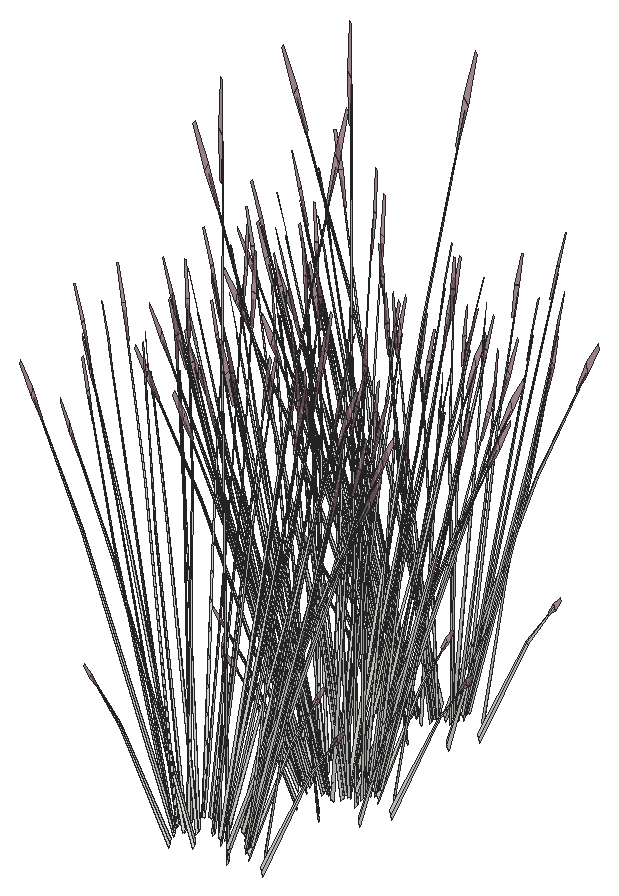
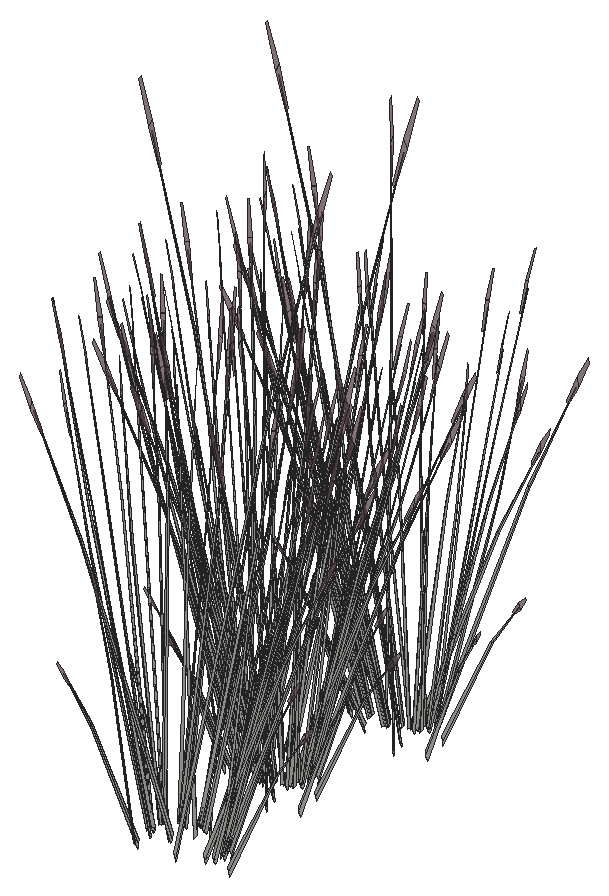
# SketchUp Ruby script. Lengths in inches.
U = 1.inch
M = Sketchup.active_model
def pt(a) = Geom::Point3d.new(a.map { |v| v * U })
def face(e, loops, mat)
  f = e.add_face(loops[0].map { |a| pt(a) })
  loops[1..].each { |l| e.add_face(l.map { |a| pt(a) }).erase! }
  f.material = f.back_material = mat if mat
  f
end
# faces: each face lists its corners as indices into pts; further lists are holes
def faces(e, pts, list, mat = nil) = list.each { |f| face(e, (f[0].is_a?(Array) ? f : [f]).map { |l| l.map { |i| pts[i] } }, mat) }
# xy, xz, yz: faces in a plane at the given z, y or x. An outline is a flat list of corners, or four numbers for a rectangle; further outlines are holes
def ring(l) = l.size == 4 ? [[l[0], l[1]], [l[2], l[1]], [l[2], l[3]], [l[0], l[3]]] : l.each_slice(2).to_a
def flat(e, list, mat, &to3) = list.each { |f| face(e, (f[0].is_a?(Array) ? f : [f]).map { |l| ring(l).map { |u, v| to3.(u, v) } }, mat) }
def xy(e, z, list, mat = nil) = flat(e, list, mat) { |x, y| [x, y, z] }
def xz(e, y, list, mat = nil) = flat(e, list, mat) { |x, z| [x, y, z] }
def yz(e, x, list, mat = nil) = flat(e, list, mat) { |y, z| [x, y, z] }
def lines(e, pts, list) = list.each { |a, b| e.add_line(pt(pts[a]), pt(pts[b])) }
# prism: a flat outline (further loops are holes) pulled along v
def prism(e, loops, v, mat = nil)
  f = face(e, loops, mat); d = Geom::Vector3d.new(v.map { |x| x * U })
  f.pushpull(f.normal.samedirection?(d) ? d.length : -d.length)
end
def box(e, o, s, mat = nil) = prism(e, [[o, [o[0] + s[0], o[1], o[2]], [o[0] + s[0], o[1] + s[1], o[2]], [o[0], o[1] + s[1], o[2]]]], [0, 0, s[2]], mat)
def at(x, y, z, deg = 0) = Geom::Transformation.translation(pt([x, y, z])) * Geom::Transformation.rotation(ORIGIN, Z_AXIS, deg.degrees)
def axes(o, x, y, z) = Geom::Transformation.new([*x, 0, *y, 0, *z, 0, *pt(o).to_a, 1])
def part(name) = M.definitions.add(name)
# library, detail: a bought-in or finely detailed component or shape, given as its bounding box
def library(name, o, s) = part(name).tap { |d| box(d.entities, o, s) }
def detail(e, o, s) = box(e.add_group.entities, o, s)
def put(e, d, t, mat = nil) = e.add_instance(d, t).tap { |i| i.material = mat if mat }
def group(e, t, mat = nil) = e.add_group.tap { |g| g.transformation = t; g.material = mat if mat }.entities
root = M.entities
M.materials.add("LightPink_Translucent").color = [144, 107, 117]
M.materials["LightPink_Translucent"].alpha = 0.75
c1 = part("blade")
p = [[2.15,0.21,22],[0,0.17,0],[0.09,0.45,0],[2.18,0.31,22],[2.29,0.31,22],[0.38,0.45,0],
  [2.48,0.24,33],[2.49,0.24,33],[2.48,0.22,33]]
faces(c1.entities,p,[[0,1,2,3],[4,5,2,3],[6,3,4,7],[8,0,3,6]])
c2 = part("seeds")
p = [[0.3,-0.1,1.38],[-0.01,-0.03,1.59],[-0.01,-0.03,0.03],[0.14,-0.07,-0.07],[0.29,-0.03,3],[0.15,0.01,3.11]]
faces(c2.entities,p,[[0,1,2,3],[1,0,4,5]],"LightPink_Translucent")
c3 = part("blade with seeds")
put(c3.entities,c1,at(0,0,0))
put(c3.entities,c2,axes([2.4,0.25,30.99],[1.5799,-0.05474,1.17369],[-0.12525,1.92788,0.29478],[-0.07173,-0.02425,1.56792]))
put(root,c3,axes([331.16,423.04,50.44],[0.32236,-0.02796,1.01491],[-0.20448,0.24636,0.74569],[-0.1593,-0.03696,0.22354]))
put(root,c3,axes([332.18,422.42,52.45],[-0.02704,0.39739,-0.10745],[-0.51189,-0.01086,-0.59638],[-0.19715,-0.0276,0.90619]))
put(root,c3,axes([336.01,423.95,52.45],[-0.25405,-0.35383,-0.10745],[0.45089,-0.17388,-0.59638],[0.19001,-0.04668,0.90619]))
put(root,c3,axes([335.98,423.64,52.14],[0.13679,-0.35544,-0.45151],[0.46898,0.12183,-0.34973],[0.18882,-0.03259,0.86392]))
put(root,c3,axes([331.52,422.97,51.43],[0.20943,-0.00885,1.51428],[-0.13893,0.38357,0.12244],[-0.29846,-0.02372,0.64734]))
put(root,c3,axes([335.9,423.77,52.4],[0.44368,-0.17257,-0.62776],[0.24726,0.35524,0.07576],[0.21437,-0.04035,0.88802]))
put(root,c3,axes([336.27,423.8,52],[0.41962,0.10901,-0.31292],[-0.12239,0.31802,0.40398],[0.16894,-0.02916,0.77298]))
put(root,c3,axes([331.34,423.3,52],[-0.41962,-0.10901,-0.31292],[0.12239,-0.31802,0.40398],[-0.16894,0.02916,0.77298]))
put(root,c3,axes([335.13,423.41,51.43],[-0.20943,0.00885,1.51428],[0.13893,-0.38357,0.12244],[0.29846,0.02372,0.64734]))
put(root,c3,axes([332.62,423.25,50.95],[0.14352,-0.05653,1.56454],[0.04949,0.39467,0.12244],[-0.31087,0.05237,0.55918]))
put(root,c3,axes([337.16,423.87,50.44],[-0.31197,0.06451,1.01491],[0.14684,-0.26661,0.74569],[0.1655,0.01824,0.22354]))
put(root,c3,axes([331.63,423.46,52.14],[-0.13679,0.35544,-0.45151],[-0.46898,-0.12183,-0.34973],[-0.18882,0.03259,0.86392]))
put(root,c3,axes([331.61,423.16,52.45],[0.25405,0.35383,-0.10745],[-0.45089,0.17388,-0.59638],[-0.19001,0.04668,0.90619]))
put(root,c3,axes([336.62,424.69,51.47],[-0.09664,-0.32847,-0.03085],[0.45676,-0.07551,-0.13989],[0.09538,0.02082,0.4614]))
put(root,c3,axes([335.4375,424.68,52.45],[0.02704,-0.39739,-0.10745],[0.51189,0.01086,-0.59638],[0.19715,0.0276,0.90619]))
put(root,c3,axes([331.61,423.64,51.43],[0.17519,-0.08265,1.51428],[0.14749,0.38193,0.12244],[-0.27504,0.08632,0.64734]))
put(root,c3,axes([335.46,424.49,52.4],[0.50473,0.00941,-0.62776],[-0.0339,0.39618,0.07576],[0.21383,0.04181,0.88802]))
put(root,c3,axes([330.7,424.98,50.44],[0.21042,-0.1771,1.01491],[0.08303,0.28036,0.74569],[-0.15207,0.0502,0.22354]))
put(root,c3,axes([335.77,424.65,52],[0.28729,0.24465,-0.31292],[-0.32804,0.23159,0.40398],[0.16667,0.03524,0.77298]))
put(root,c3,axes([331.49,424.22,52],[-0.43951,0.05584,-0.31292],[-0.11606,-0.31924,0.40398],[-0.12595,0.08575,0.77298]))
put(root,c3,axes([334.73,424.03,51.43],[-0.18755,-0.06732,1.51428],[0.38813,-0.28243,0.12244],[0.24191,0.12741,0.64734]))
put(root,c3,axes([334.77,423.14,51.95],[-0.4363,-0.20303,1.22187],[0.46069,-0.31611,0.5272],[0.14077,0.1905,1.18105]))
put(root,c3,axes([331.625,424,52.45],[0.46706,0.21546,-0.10745],[-0.26908,0.31203,-0.59638],[-0.13196,0.10846,0.90619]))
put(root,c3,axes([335.43,424.79,50.44],[-0.28429,-0.11236,1.01491],[0.36709,-0.11416,0.74569],[0.09901,0.0967,0.22354]))
put(root,c3,axes([334.43,425.11,52.45],[0.30087,-0.33447,-0.10745],[0.43572,0.19269,-0.59638],[0.15146,0.0945,0.90619]))
put(root,c3,axes([332.25,423.9,51.43],[0.12611,-0.12006,1.51428],[0.31843,0.32408,0.12244],[-0.2184,0.14759,0.64734]))
put(root,c3,axes([331.86,424.25,52.14],[0.12971,0.3568,-0.45151],[-0.49122,0.06241,-0.34973],[-0.14077,0.09583,0.86392]))
put(root,c3,axes([334.74,423.53,50.51],[-0.01379,-0.36791,1.24828],[0.62424,0.09537,0.52853],[-0.14764,0.20132,1.17828]))
put(root,c3,axes([334.79,424.95,52.14],[0.49824,-0.09289,-0.45151],[0.08716,0.35177,-0.34973],[0.13382,0.10081,0.86392]))
put(root,c3,axes([332.16,424.2,51.43],[0.09401,-0.13431,1.51428],[0.3944,0.27795,0.12244],[-0.17792,0.17323,0.64734]))
put(root,c3,axes([332.27,424.95,52],[-0.34164,0.20573,-0.31292],[-0.3234,-0.23491,0.40398],[-0.04921,0.11936,0.77298]))
put(root,c3,axes([333.25,425.13,52.45],[0.49409,-0.18193,-0.10745],[0.24281,0.32289,-0.59638],[0.06519,0.13607,0.90619]))
put(root,c3,axes([332.48,425.75,50.44],[-0.01307,-0.23234,1.01491],[0.32652,0.16572,0.74569],[-0.06422,0.11074,0.22354]))
put(root,c3,axes([332.61,424.86,52.42],[0.36145,0.26255,-0.50118],[-0.38183,0.22994,-0.3882],[-0.055,0.1334,0.95895]))
put(root,c3,axes([333.68,425.11,52.14],[0.49634,0.09796,-0.45151],[-0.17013,0.33585,-0.34973],[0.04551,0.13522,0.86392]))
put(root,c3,axes([333.96,424.42,51.43],[-0.11542,-0.12546,1.51428],[0.53333,-0.10562,0.12244],[0.12054,0.19696,0.64734]))
put(root,c3,axes([333.45,425.32,52],[-0.15222,0.30049,-0.31292],[-0.44409,-0.08764,0.40398],[0.04072,0.12098,0.77298]))
put(root,c3,axes([332.49,424.74,52.72],[-0.01314,0.36145,-0.69681],[-0.55324,-0.02428,0.08409],[-0.05838,0.15313,0.9857]))
put(root,c3,axes([334.28,431.48,51.43],[0.11542,0.12546,1.51428],[-0.53333,0.10562,0.12244],[-0.12054,-0.19696,0.64734]))
put(root,c3,axes([333.02,424.48,51.43],[-0.01236,-0.14998,1.51428],[0.53562,0.09949,0.12244],[-0.03313,0.21373,0.64734]))
put(root,c3,axes([335.7,431.57,52.4],[-0.24099,-0.31773,-0.62776],[0.49607,-0.17707,0.07576],[-0.05635,-0.15352,0.88802]))
put(root,c3,axes([333.5,425.05,52.4],[0.24099,0.31773,-0.62776],[-0.49607,0.17707,0.07576],[0.05635,0.15352,0.88802]))
put(root,c3,axes([336.7,431.88,52.4],[0.01314,-0.36145,-0.62776],[0.55324,0.02428,0.07576],[0.05838,-0.15313,0.88802]))
put(root,c3,axes([335.75,431.3,52],[0.15222,-0.30049,-0.31292],[0.44409,0.08764,0.40398],[-0.04072,-0.12098,0.77298]))
put(root,c3,axes([336.08,431.7,51.43],[-0.09401,0.13431,1.51428],[-0.3944,-0.27795,0.12244],[0.17792,-0.17323,0.64734]))
put(root,c3,axes([335.52,431.51,52.14],[-0.49634,-0.09796,-0.45151],[0.17013,-0.33585,-0.34973],[-0.04551,-0.13522,0.86392]))
put(root,c3,axes([335.83,430.67,50.44],[0.06477,0.22786,1.01491],[-0.35932,-0.1262,0.74569],[0.03867,-0.11667,0.22354]))
put(root,c3,axes([332.31,425.25,50.97],[0.01109,-0.20172,1.3638],[0.49896,0.10655,0.18846],[-0.04323,0.21498,0.64398]))
put(root,c3,axes([336.59,431.76,52.14],[-0.36145,-0.26255,-0.45151],[0.38183,-0.22994,-0.34973],[0.055,-0.1334,0.86392]))
put(root,c3,axes([335.95,431.49,52.45],[-0.49409,0.18193,-0.10745],[-0.24281,-0.32289,-0.59638],[-0.06519,-0.13607,0.90619]))
put(root,c3,axes([336.97,431.9,52.45],[-0.55492,-0.01936,-0.10745],[0.01517,-0.36657,-0.59638],[0.03855,-0.14118,0.90619]))
put(root,c3,axes([336.93,431.67,52],[0.34164,-0.20573,-0.31292],[0.3234,0.23491,0.40398],[0.04921,-0.11936,0.77298]))
put(root,c3,axes([333.98,430.94,50.44],[0.26338,0.136,1.01491],[-0.38358,0.08175,0.74569],[-0.08207,-0.10452,0.22354]))
put(root,c3,axes([334.62,431.66,52.4],[-0.43054,-0.18887,-0.62776],[0.30598,-0.33097,0.07576],[-0.15599,-0.11277,0.88802]))
put(root,c3,axes([334.47,431.41,52],[-0.07798,-0.31474,-0.31292],[0.44579,-0.08311,0.40398],[-0.11974,-0.09019,0.77298]))
put(root,c3,axes([333.51,431.87,51.43],[0.18755,0.06732,1.51428],[-0.38813,0.28243,0.12244],[-0.24191,-0.12741,0.64734]))
put(root,c3,axes([334.41,431.67,52.14],[-0.49824,0.09289,-0.45151],[-0.08716,-0.35177,-0.34973],[-0.13382,-0.10081,0.86392]))
put(root,c3,axes([337.36,432.51,52.4],[0.26374,-0.30832,-0.62776],[0.46217,0.21911,0.07576],[0.15748,-0.11171,0.88802]))
put(root,c3,axes([337.34,432.37,52.14],[-0.12971,-0.3568,-0.45151],[0.49122,-0.06241,-0.34973],[0.14077,-0.09583,0.86392]))
put(root,c3,axes([337.58,432.625,52.45],[-0.46706,-0.21546,-0.10745],[0.26908,-0.31203,-0.59638],[0.13196,-0.10846,0.90619]))
put(root,c3,axes([335.65,433.8,50.9375],[0.43633,0.15757,1.33654],[-0.42745,0.33945,0.52853],[-0.19146,-0.20119,1.12046]))
put(root,c3,axes([337.95,431.66,50.44],[-0.16818,0.19891,1.01491],[-0.14456,-0.26725,0.74569],[0.1389,-0.06697,0.22354]))
put(root,c3,axes([337.71,432.41,52],[0.43951,-0.05584,-0.31292],[0.11606,0.31924,0.40398],[0.12595,-0.08575,0.77298]))
put(root,c3,axes([333.43,431.97,52],[-0.28729,-0.24465,-0.31292],[0.32804,-0.23159,0.40398],[-0.16667,-0.03524,0.77298]))
put(root,c3,axes([333.74,432.13,52.4],[-0.50473,-0.00941,-0.62776],[0.0339,-0.39618,0.07576],[-0.21383,-0.04181,0.88802]))
put(root,c3,axes([333.57,432.21,52.14],[-0.36663,0.25884,-0.45151],[-0.32109,-0.27343,-0.34973],[-0.18628,-0.03938,0.86392]))
put(root,c3,axes([332.74,432.55,50.44],[0.32236,-0.02796,1.01491],[-0.20448,0.24636,0.74569],[-0.1593,-0.03696,0.22354]))
put(root,c3,axes([333.76,431.94,52.45],[-0.02704,0.39739,-0.10745],[-0.51189,-0.01086,-0.59638],[-0.19715,-0.0276,0.90619]))
put(root,c3,axes([337.59,433.47,52.45],[-0.25405,-0.35383,-0.10745],[0.45089,-0.17388,-0.59638],[0.19001,-0.04668,0.90619]))
put(root,c3,axes([337.57,433.16,52.14],[0.13679,-0.35544,-0.45151],[0.46898,0.12183,-0.34973],[0.18882,-0.03259,0.86392]))
put(root,c3,axes([333.11,432.49,51.43],[0.20943,-0.00885,1.51428],[-0.13893,0.38357,0.12244],[-0.29846,-0.02372,0.64734]))
put(root,c3,axes([337.48,433.29,52.4],[0.44368,-0.17257,-0.62776],[0.24726,0.35524,0.07576],[0.21437,-0.04035,0.88802]))
put(root,c3,axes([337.86,433.32,52],[0.41962,0.10901,-0.31292],[-0.12239,0.31802,0.40398],[0.16894,-0.02916,0.77298]))
put(root,c3,axes([332.93,432.82,52],[-0.41962,-0.10901,-0.31292],[0.12239,-0.31802,0.40398],[-0.16894,0.02916,0.77298]))
put(root,c3,axes([336.72,432.93,51.43],[-0.20943,0.00885,1.51428],[0.13893,-0.38357,0.12244],[0.29846,0.02372,0.64734]))
put(root,c3,axes([334.21,432.76,50.95],[0.14352,-0.05653,1.56454],[0.04949,0.39467,0.12244],[-0.31087,0.05237,0.55918]))
put(root,c3,axes([338.75,433.39,50.44],[-0.31197,0.06451,1.01491],[0.14684,-0.26661,0.74569],[0.1655,0.01824,0.22354]))
put(root,c3,axes([333.22,432.98,52.14],[-0.13679,0.35544,-0.45151],[-0.46898,-0.12183,-0.34973],[-0.18882,0.03259,0.86392]))
put(root,c3,axes([333.19,432.68,52.45],[0.25405,0.35383,-0.10745],[-0.45089,0.17388,-0.59638],[-0.19001,0.04668,0.90619]))
put(root,c3,axes([338.21,434.21,51.47],[-0.09664,-0.32847,-0.03085],[0.45676,-0.07551,-0.13989],[0.09538,0.02082,0.4614]))
put(root,c3,axes([337.02,434.2,52.45],[0.02704,-0.39739,-0.10745],[0.51189,0.01086,-0.59638],[0.19715,0.0276,0.90619]))
put(root,c3,axes([333.2,433.16,51.43],[0.17519,-0.08265,1.51428],[0.14749,0.38193,0.12244],[-0.27504,0.08632,0.64734]))
put(root,c3,axes([337.05,434.01,52.4],[0.50473,0.00941,-0.62776],[-0.0339,0.39618,0.07576],[0.21383,0.04181,0.88802]))
put(root,c3,axes([332.29,434.5,50.44],[0.21042,-0.1771,1.01491],[0.08303,0.28036,0.74569],[-0.15207,0.0502,0.22354]))
put(root,c3,axes([337.35,434.17,52],[0.28729,0.24465,-0.31292],[-0.32804,0.23159,0.40398],[0.16667,0.03524,0.77298]))
put(root,c3,axes([333.08,433.73,52],[-0.43951,0.05584,-0.31292],[-0.11606,-0.31924,0.40398],[-0.12595,0.08575,0.77298]))
put(root,c3,axes([336.32,433.55,51.43],[-0.18755,-0.06732,1.51428],[0.38813,-0.28243,0.12244],[0.24191,0.12741,0.64734]))
put(root,c3,axes([336.36,432.66,51.95],[-0.4363,-0.20303,1.22187],[0.46069,-0.31611,0.5272],[0.14077,0.1905,1.18105]))
put(root,c3,axes([333.21,433.52,52.45],[0.46706,0.21546,-0.10745],[-0.26908,0.31203,-0.59638],[-0.13196,0.10846,0.90619]))
put(root,c3,axes([337.01,434.3125,50.44],[-0.28429,-0.11236,1.01491],[0.36709,-0.11416,0.74569],[0.09901,0.0967,0.22354]))
put(root,c3,axes([336.02,434.63,52.45],[0.30087,-0.33447,-0.10745],[0.43572,0.19269,-0.59638],[0.15146,0.0945,0.90619]))
put(root,c3,axes([333.84,433.42,51.43],[0.12611,-0.12006,1.51428],[0.31843,0.32408,0.12244],[-0.2184,0.14759,0.64734]))
put(root,c3,axes([333.44,433.77,52.14],[0.12971,0.3568,-0.45151],[-0.49122,0.06241,-0.34973],[-0.14077,0.09583,0.86392]))
put(root,c3,axes([336.32,433.05,50.51],[-0.01379,-0.36791,1.24828],[0.62424,0.09537,0.52853],[-0.14764,0.20132,1.17828]))
put(root,c3,axes([336.37,434.47,52.14],[0.49824,-0.09289,-0.45151],[0.08716,0.35177,-0.34973],[0.13382,0.10081,0.86392]))
put(root,c3,axes([333.75,433.72,51.43],[0.09401,-0.13431,1.51428],[0.3944,0.27795,0.12244],[-0.17792,0.17323,0.64734]))
put(root,c3,axes([333.85,434.47,52],[-0.34164,0.20573,-0.31292],[-0.3234,-0.23491,0.40398],[-0.04921,0.11936,0.77298]))
put(root,c3,axes([334.84,434.65,52.45],[0.49409,-0.18193,-0.10745],[0.24281,0.32289,-0.59638],[0.06519,0.13607,0.90619]))
put(root,c3,axes([334.07,435.27,50.44],[-0.01307,-0.23234,1.01491],[0.32652,0.16572,0.74569],[-0.06422,0.11074,0.22354]))
put(root,c3,axes([334.19,434.375,52.42],[0.36145,0.26255,-0.50118],[-0.38183,0.22994,-0.3882],[-0.055,0.1334,0.95895]))
put(root,c3,axes([335.27,434.63,52.14],[0.49634,0.09796,-0.45151],[-0.17013,0.33585,-0.34973],[0.04551,0.13522,0.86392]))
put(root,c3,axes([335.55,433.9375,51.43],[-0.11542,-0.12546,1.51428],[0.53333,-0.10562,0.12244],[0.12054,0.19696,0.64734]))
put(root,c3,axes([335.04,434.84,52],[-0.15222,0.30049,-0.31292],[-0.44409,-0.08764,0.40398],[0.04072,0.12098,0.77298]))
put(root,c3,axes([334.08,434.26,52.72],[-0.01314,0.36145,-0.69681],[-0.55324,-0.02428,0.08409],[-0.05838,0.15313,0.9857]))
put(root,c3,axes([334.61,434,51.43],[-0.01236,-0.14998,1.51428],[0.53562,0.09949,0.12244],[-0.03313,0.21373,0.64734]))
put(root,c3,axes([335.09,434.57,52.4],[0.24099,0.31773,-0.62776],[-0.49607,0.17707,0.07576],[0.05635,0.15352,0.88802]))
put(root,c3,axes([332.69,441.35,51.43],[0.11542,0.12546,1.51428],[-0.53333,0.10562,0.12244],[-0.12054,-0.19696,0.64734]))
put(root,c3,axes([334.11,441.44,52.4],[-0.24099,-0.31773,-0.62776],[0.49607,-0.17707,0.07576],[-0.05635,-0.15352,0.88802]))
put(root,c3,axes([333.9,434.76,50.97],[0.01109,-0.20172,1.3638],[0.49896,0.10655,0.18846],[-0.04323,0.21498,0.64398]))
put(root,c3,axes([335.12,441.75,52.4],[0.01314,-0.36145,-0.62776],[0.55324,0.02428,0.07576],[0.05838,-0.15313,0.88802]))
put(root,c3,axes([334.16,441.17,52],[0.15222,-0.30049,-0.31292],[0.44409,0.08764,0.40398],[-0.04072,-0.12098,0.77298]))
put(root,c3,axes([334.5,441.57,51.43],[-0.09401,0.13431,1.51428],[-0.3944,-0.27795,0.12244],[0.17792,-0.17323,0.64734]))
put(root,c3,axes([333.93,441.38,52.14],[-0.49634,-0.09796,-0.45151],[0.17013,-0.33585,-0.34973],[-0.04551,-0.13522,0.86392]))
put(root,c3,axes([334.24,440.54,50.44],[0.06477,0.22786,1.01491],[-0.35932,-0.1262,0.74569],[0.03867,-0.11667,0.22354]))
put(root,c3,axes([335.01,441.63,52.14],[-0.36145,-0.26255,-0.45151],[0.38183,-0.22994,-0.34973],[0.055,-0.1334,0.86392]))
put(root,c3,axes([334.36,441.36,52.45],[-0.49409,0.18193,-0.10745],[-0.24281,-0.32289,-0.59638],[-0.06519,-0.13607,0.90619]))
put(root,c3,axes([335.38,441.77,52.45],[-0.55492,-0.01936,-0.10745],[0.01517,-0.36657,-0.59638],[0.03855,-0.14118,0.90619]))
put(root,c3,axes([335.35,441.53,52],[0.34164,-0.20573,-0.31292],[0.3234,0.23491,0.40398],[0.04921,-0.11936,0.77298]))
put(root,c3,axes([332.39,440.81,50.44],[0.26338,0.136,1.01491],[-0.38358,0.08175,0.74569],[-0.08207,-0.10452,0.22354]))
put(root,c3,axes([333.03,441.53,52.4],[-0.43054,-0.18887,-0.62776],[0.30598,-0.33097,0.07576],[-0.15599,-0.11277,0.88802]))
put(root,c3,axes([332.88,441.28,52],[-0.07798,-0.31474,-0.31292],[0.44579,-0.08311,0.40398],[-0.11974,-0.09019,0.77298]))
put(root,c3,axes([331.92,441.74,51.43],[0.18755,0.06732,1.51428],[-0.38813,0.28243,0.12244],[-0.24191,-0.12741,0.64734]))
put(root,c3,axes([332.83,441.54,52.14],[-0.49824,0.09289,-0.45151],[-0.08716,-0.35177,-0.34973],[-0.13382,-0.10081,0.86392]))
put(root,c3,axes([335.77,442.38,52.4],[0.26374,-0.30832,-0.62776],[0.46217,0.21911,0.07576],[0.15748,-0.11171,0.88802]))
put(root,c3,axes([335.76,442.24,52.14],[-0.12971,-0.3568,-0.45151],[0.49122,-0.06241,-0.34973],[0.14077,-0.09583,0.86392]))
put(root,c3,axes([335.99,442.49,52.45],[-0.46706,-0.21546,-0.10745],[0.26908,-0.31203,-0.59638],[0.13196,-0.10846,0.90619]))
put(root,c3,axes([334.06,443.67,50.9375],[0.43633,0.15757,1.33654],[-0.42745,0.33945,0.52853],[-0.19146,-0.20119,1.12046]))
put(root,c3,axes([336.36,441.53,50.44],[-0.16818,0.19891,1.01491],[-0.14456,-0.26725,0.74569],[0.1389,-0.06697,0.22354]))
put(root,c3,axes([336.12,442.27,52],[0.43951,-0.05584,-0.31292],[0.11606,0.31924,0.40398],[0.12595,-0.08575,0.77298]))
put(root,c3,axes([331.85,441.83,52],[-0.28729,-0.24465,-0.31292],[0.32804,-0.23159,0.40398],[-0.16667,-0.03524,0.77298]))
put(root,c3,axes([332.15,442,52.4],[-0.50473,-0.00941,-0.62776],[0.0339,-0.39618,0.07576],[-0.21383,-0.04181,0.88802]))
put(root,c3,axes([331.98,442.08,52.14],[-0.36663,0.25884,-0.45151],[-0.32109,-0.27343,-0.34973],[-0.18628,-0.03938,0.86392]))
put(root,c3,axes([331.16,442.42,50.44],[0.32236,-0.02796,1.01491],[-0.20448,0.24636,0.74569],[-0.1593,-0.03696,0.22354]))
put(root,c3,axes([332.18,441.81,52.45],[-0.02704,0.39739,-0.10745],[-0.51189,-0.01086,-0.59638],[-0.19715,-0.0276,0.90619]))
put(root,c3,axes([336.01,443.33,52.45],[-0.25405,-0.35383,-0.10745],[0.45089,-0.17388,-0.59638],[0.19001,-0.04668,0.90619]))
put(root,c3,axes([335.98,443.03,52.14],[0.13679,-0.35544,-0.45151],[0.46898,0.12183,-0.34973],[0.18882,-0.03259,0.86392]))
put(root,c3,axes([331.52,442.35,51.43],[0.20943,-0.00885,1.51428],[-0.13893,0.38357,0.12244],[-0.29846,-0.02372,0.64734]))
put(root,c3,axes([335.9,443.16,52.4],[0.44368,-0.17257,-0.62776],[0.24726,0.35524,0.07576],[0.21437,-0.04035,0.88802]))
put(root,c3,axes([336.27,443.19,52],[0.41962,0.10901,-0.31292],[-0.12239,0.31802,0.40398],[0.16894,-0.02916,0.77298]))
put(root,c3,axes([331.34,442.68,52],[-0.41962,-0.10901,-0.31292],[0.12239,-0.31802,0.40398],[-0.16894,0.02916,0.77298]))
put(root,c3,axes([335.13,442.8,51.43],[-0.20943,0.00885,1.51428],[0.13893,-0.38357,0.12244],[0.29846,0.02372,0.64734]))
put(root,c3,axes([332.62,442.63,50.95],[0.14352,-0.05653,1.56454],[0.04949,0.39467,0.12244],[-0.31087,0.05237,0.55918]))
put(root,c3,axes([337.16,443.26,50.44],[-0.31197,0.06451,1.01491],[0.14684,-0.26661,0.74569],[0.1655,0.01824,0.22354]))
put(root,c3,axes([331.63,442.85,52.14],[-0.13679,0.35544,-0.45151],[-0.46898,-0.12183,-0.34973],[-0.18882,0.03259,0.86392]))
put(root,c3,axes([331.61,442.54,52.45],[0.25405,0.35383,-0.10745],[-0.45089,0.17388,-0.59638],[-0.19001,0.04668,0.90619]))
put(root,c3,axes([336.62,444.08,51.47],[-0.09664,-0.32847,-0.03085],[0.45676,-0.07551,-0.13989],[0.09538,0.02082,0.4614]))
put(root,c3,axes([335.4375,444.07,52.45],[0.02704,-0.39739,-0.10745],[0.51189,0.01086,-0.59638],[0.19715,0.0276,0.90619]))
put(root,c3,axes([331.61,443.03,51.43],[0.17519,-0.08265,1.51428],[0.14749,0.38193,0.12244],[-0.27504,0.08632,0.64734]))
